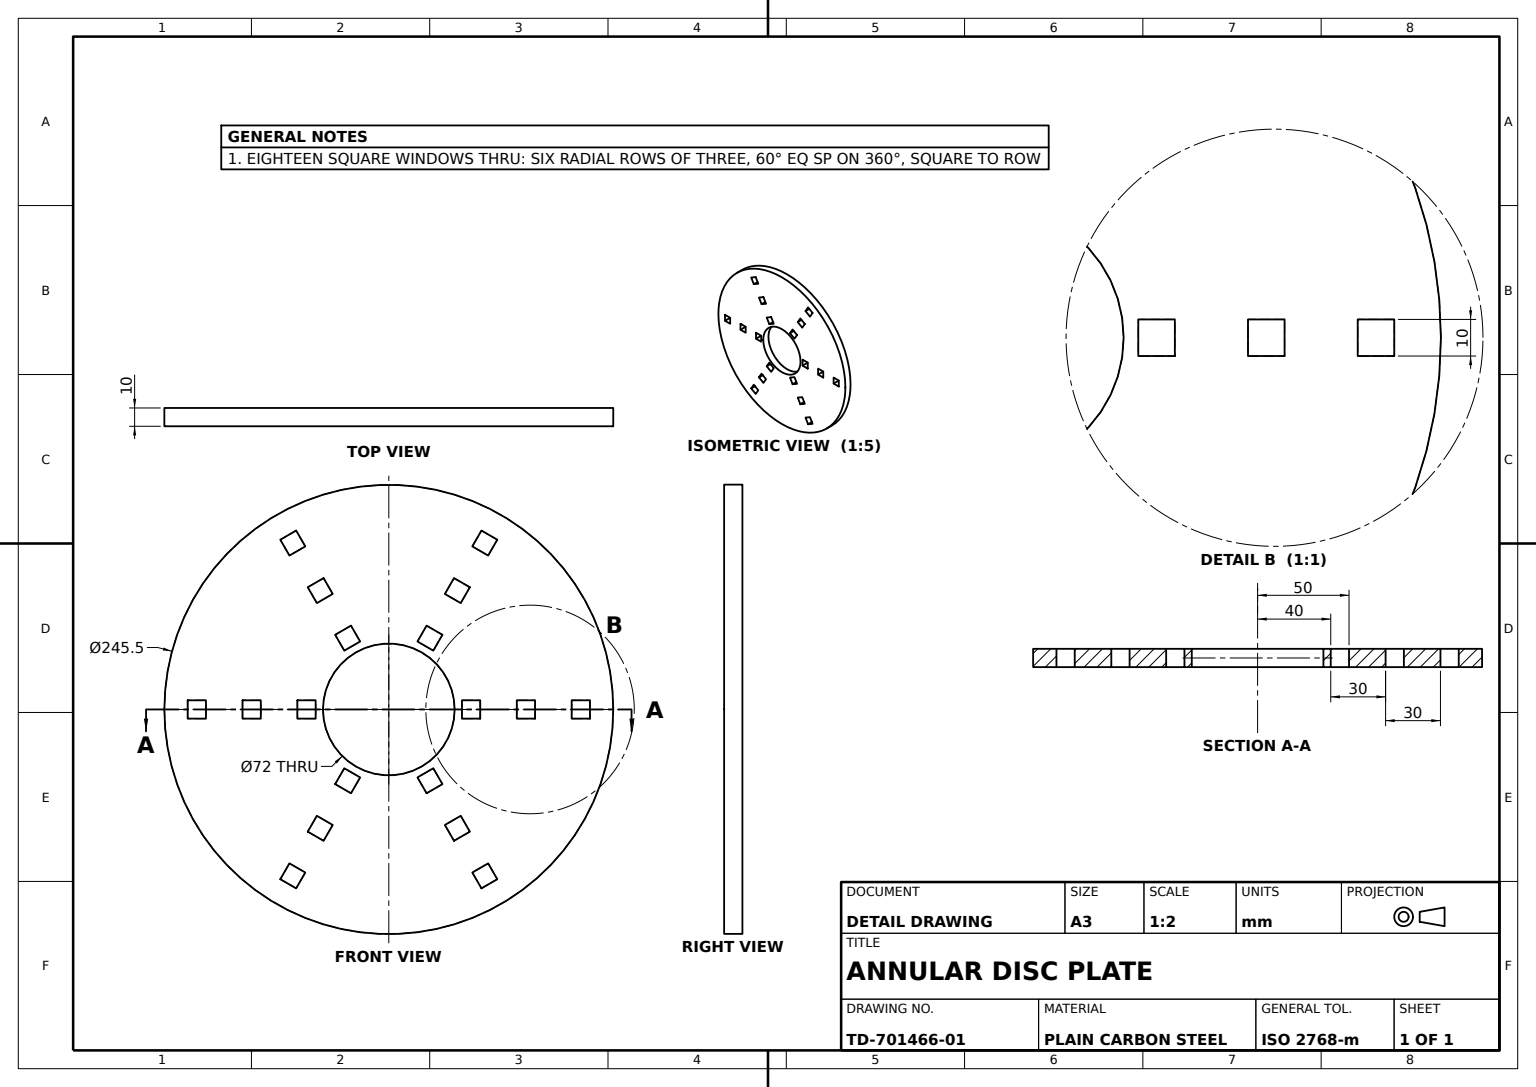
solid
v1 (54.330127,84.10254,10)
v2 (59.330127,92.762794,10)
e1 v1 v2 LINE
v3 (59.330127,92.762794,0)
e2 v3 v2 LINE
v4 (54.330127,84.10254,0)
e3 v4 v3 LINE
e4 v4 v1 LINE
face PLANE(AX(P(34.330127,49.461524,0),D(0.866025404,-0.5,0),D(0.5,0.866025404,0))) rev [e1 -e2 -e3 e4]
v5 (39.330127,-58.121778,0)
v6 (39.330127,-58.121778,10)
e5 v5 v6 LINE
v7 (30.669873,-63.121778,10)
e6 v7 v6 LINE
v8 (30.669873,-63.121778,0)
e7 v8 v7 LINE
e8 v8 v5 LINE
face PLANE(AX(P(35,-60.621778,0),D(0.5,-0.866025404,0),D(0.866025404,0.5,0))) [e5 -e6 -e7 e8]
v9 (29.330127,40.80127,0)
v10 (20.669873,45.80127,0)
e9 v9 v10 LINE
v11 (29.330127,40.80127,10)
e10 v9 v11 LINE
v12 (20.669873,45.80127,10)
e11 v11 v12 LINE
e12 v10 v12 LINE
face PLANE(AX(P(25,43.30127,0),D(0.5,0.866025404,0),D(-0.866025404,0.5,0))) rev [-e9 e10 e11 -e12]
v13 (-54.330127,-84.10254,0)
v14 (-45.669873,-89.10254,0)
e13 v13 v14 LINE
v15 (-45.669873,-89.10254,10)
e14 v14 v15 LINE
v16 (-54.330127,-84.10254,10)
e15 v16 v15 LINE
e16 v13 v16 LINE
face PLANE(AX(P(-50,-86.60254,0),D(-0.5,-0.866025404,0),D(0.866025404,-0.5,0))) [e13 e14 -e15 -e16]
v17 (122.75,0,10)
v18 (-122.75,0,10)
e17 v17 v18 CIRCLE(AX(P(0,0,10),D(0,0,1),D(1,0,0)),122.75)
e18 v18 v17 CIRCLE(AX(P(0,0,10),D(0,0,1),D(1,0,0)),122.75)
v19 (-15.669873,37.141016,10)
v20 (-24.330127,32.141016,10)
e19 v19 v20 LINE
v21 (-29.330127,40.80127,10)
e20 v21 v20 LINE
v22 (-20.669873,45.80127,10)
e21 v22 v21 LINE
e22 v19 v22 LINE
v23 (44.330127,66.782032,10)
v24 (35.669873,71.782032,10)
e23 v23 v24 LINE
v25 (39.330127,58.121778,10)
e24 v25 v23 LINE
v26 (30.669873,63.121778,10)
e25 v25 v26 LINE
e26 v24 v26 LINE
v27 (24.330127,32.141016,10)
e27 v27 v11 LINE
v28 (15.669873,37.141016,10)
e28 v27 v28 LINE
e29 v12 v28 LINE
v29 (-24.330127,-32.141016,10)
v30 (-15.669873,-37.141016,10)
e30 v29 v30 LINE
v31 (-20.669873,-45.80127,10)
e31 v31 v30 LINE
v32 (-29.330127,-40.80127,10)
e32 v32 v31 LINE
e33 v29 v32 LINE
v33 (-40,5,10)
v34 (-50,5,10)
e34 v33 v34 LINE
v35 (-40,-5,10)
e35 v33 v35 LINE
v36 (-50,-5,10)
e36 v36 v35 LINE
e37 v34 v36 LINE
v37 (29.330127,-40.80127,10)
v38 (24.330127,-32.141016,10)
e38 v37 v38 LINE
v39 (20.669873,-45.80127,10)
e39 v39 v37 LINE
v40 (15.669873,-37.141016,10)
e40 v40 v39 LINE
e41 v40 v38 LINE
v41 (35.669873,-71.782032,10)
e42 v7 v41 LINE
v42 (44.330127,-66.782032,10)
e43 v42 v6 LINE
e44 v41 v42 LINE
v43 (-50.669873,-97.762794,10)
e45 v43 v15 LINE
v44 (-59.330127,-92.762794,10)
e46 v44 v43 LINE
e47 v16 v44 LINE
v45 (50,5,10)
v46 (40,5,10)
e48 v45 v46 LINE
v47 (50,-5,10)
e49 v47 v45 LINE
v48 (40,-5,10)
e50 v48 v47 LINE
e51 v48 v46 LINE
v49 (-44.330127,66.782032,10)
v50 (-39.330127,58.121778,10)
e52 v49 v50 LINE
v51 (-35.669873,71.782032,10)
e53 v51 v49 LINE
v52 (-30.669873,63.121778,10)
e54 v52 v51 LINE
e55 v52 v50 LINE
v53 (-36,0,10)
v54 (36,0,10)
e56 v53 v54 CIRCLE(AX(P(0,0,10),D(0,0,1),D(1,0,0)),36)
e57 v54 v53 CIRCLE(AX(P(0,0,10),D(0,0,1),D(1,0,0)),36)
v55 (-39.330127,-58.121778,10)
v56 (-44.330127,-66.782032,10)
e58 v55 v56 LINE
v57 (-30.669873,-63.121778,10)
e59 v55 v57 LINE
v58 (-35.669873,-71.782032,10)
e60 v58 v57 LINE
e61 v56 v58 LINE
v59 (-80,5,10)
v60 (-80,-5,10)
e62 v59 v60 LINE
v61 (-70,5,10)
e63 v61 v59 LINE
v62 (-70,-5,10)
e64 v61 v62 LINE
e65 v60 v62 LINE
v63 (-59.330127,92.762794,10)
v64 (-54.330127,84.10254,10)
e66 v63 v64 LINE
v65 (-50.669873,97.762794,10)
e67 v65 v63 LINE
v66 (-45.669873,89.10254,10)
e68 v66 v65 LINE
e69 v66 v64 LINE
v67 (100,-5,10)
v68 (100,5,10)
e70 v67 v68 LINE
v69 (110,5,10)
e71 v69 v68 LINE
v70 (110,-5,10)
e72 v70 v69 LINE
e73 v67 v70 LINE
v71 (-110,5,10)
v72 (-110,-5,10)
e74 v71 v72 LINE
v73 (-100,5,10)
e75 v73 v71 LINE
v74 (-100,-5,10)
e76 v73 v74 LINE
e77 v72 v74 LINE
v75 (45.669873,-89.10254,10)
v76 (54.330127,-84.10254,10)
e78 v75 v76 LINE
v77 (59.330127,-92.762794,10)
e79 v77 v76 LINE
v78 (50.669873,-97.762794,10)
e80 v78 v77 LINE
e81 v75 v78 LINE
v79 (80,5,10)
v80 (70,5,10)
e82 v79 v80 LINE
v81 (80,-5,10)
e83 v81 v79 LINE
v82 (70,-5,10)
e84 v82 v81 LINE
e85 v82 v80 LINE
v83 (50.669873,97.762794,10)
v84 (45.669873,89.10254,10)
e86 v83 v84 LINE
e87 v2 v83 LINE
e88 v1 v84 LINE
face PLANE(AX(P(0,0,10),D(0,0,1),D(1,0,0))) [e17 e18] [e19 -e20 -e21 -e22] [-e23 -e24 e25 -e26] [-e11 -e27 e28 -e29] [e30 -e31 -e32 -e33] [-e34 e35 -e36 -e37] [-e38 -e39 -e40 e41] [-e42 e6 -e43 -e44] [-e45 -e46 -e47 e15] [-e48 -e49 -e50 e51] [-e52 -e53 -e54 e55] [-e56 -e57] [-e58 e59 -e60 -e61] [-e62 -e63 e64 -e65] [-e66 -e67 -e68 e69] [e70 -e71 -e72 -e73] [-e74 -e75 e76 -e77] [e78 -e79 -e80 -e81] [-e82 -e83 -e84 e85] [-e86 -e87 -e1 e88]
v85 (-36,0,0)
e89 v85 v53 LINE
v86 (36,0,0)
e90 v86 v54 LINE
e91 v85 v86 CIRCLE(AX(P(0,0,0),D(0,0,1),D(1,0,0)),36)
face CYL(AX(P(0,0,0),D(0,0,1),D(1,0,0)),36) rev [e89 e56 -e90 -e91]
v87 (29.330127,-40.80127,0)
e92 v87 v37 LINE
v88 (24.330127,-32.141016,0)
e93 v88 v38 LINE
e94 v87 v88 LINE
face PLANE(AX(P(4.330127,2.5,0),D(0.866025404,0.5,0),D(-0.5,0.866025404,0))) rev [e92 e38 -e93 -e94]
v89 (-35.669873,-71.782032,0)
v90 (-30.669873,-63.121778,0)
e95 v89 v90 LINE
e96 v89 v58 LINE
e97 v90 v57 LINE
face PLANE(AX(P(-10.669873,-28.480762,0),D(0.866025404,-0.5,0),D(0.5,0.866025404,0))) rev [-e95 e96 e60 -e97]
e98 v86 v85 CIRCLE(AX(P(0,0,0),D(0,0,1),D(1,0,0)),36)
face CYL(AX(P(0,0,0),D(0,0,1),D(1,0,0)),36) rev [-e98 e90 e57 -e89]
v91 (-45.669873,89.10254,0)
v92 (-50.669873,97.762794,0)
e99 v91 v92 LINE
e100 v91 v66 LINE
e101 v92 v65 LINE
face PLANE(AX(P(-25.669873,54.461524,0),D(0.866025404,0.5,0),D(-0.5,0.866025404,0))) rev [-e99 e100 e68 -e101]
v93 (35.669873,-71.782032,0)
e102 v8 v93 LINE
e103 v93 v41 LINE
face PLANE(AX(P(10.669873,-28.480762,0),D(-0.866025404,-0.5,0),D(0.5,-0.866025404,0))) rev [-e102 e7 e42 -e103]
v94 (20.669873,-45.80127,0)
e104 v94 v39 LINE
e105 v94 v87 LINE
face PLANE(AX(P(25,-43.30127,0),D(0.5,-0.866025404,0),D(0.866025404,0.5,0))) rev [e104 e39 -e92 -e105]
v95 (50,5,0)
e106 v95 v45 LINE
v96 (40,5,0)
e107 v96 v46 LINE
e108 v95 v96 LINE
face PLANE(AX(P(0,5,0),D(0,1,0),D(-1,0,0))) rev [e106 e48 -e107 -e108]
v97 (45.669873,-89.10254,0)
v98 (50.669873,-97.762794,0)
e109 v97 v98 LINE
e110 v97 v75 LINE
e111 v98 v78 LINE
face PLANE(AX(P(25.669873,-54.461524,0),D(-0.866025404,-0.5,0),D(0.5,-0.866025404,0))) rev [-e109 e110 e81 -e111]
v99 (50,-5,0)
e112 v99 v95 LINE
e113 v99 v47 LINE
face PLANE(AX(P(50,0,0),D(1,0,0),D(0,0,-1))) rev [-e106 -e112 e113 e49]
v100 (-40,-5,0)
e114 v100 v35 LINE
v101 (-50,-5,0)
e115 v101 v100 LINE
e116 v101 v36 LINE
face PLANE(AX(P(0,-5,0),D(0,-1,0),D(1,0,0))) rev [e36 -e114 -e115 e116]
v102 (35.669873,71.782032,0)
e117 v102 v24 LINE
v103 (44.330127,66.782032,0)
e118 v103 v102 LINE
e119 v103 v23 LINE
face PLANE(AX(P(40,69.282032,0),D(0.5,0.866025404,0),D(-0.866025404,0.5,0))) rev [e23 -e117 -e118 e119]
v104 (-39.330127,58.121778,0)
e120 v104 v50 LINE
v105 (-44.330127,66.782032,0)
e121 v105 v104 LINE
e122 v105 v49 LINE
face PLANE(AX(P(-19.330127,23.480762,0),D(-0.866025404,-0.5,0),D(0.5,-0.866025404,0))) rev [e52 -e120 -e121 e122]
v106 (39.330127,58.121778,0)
v107 (30.669873,63.121778,0)
e123 v106 v107 LINE
e124 v107 v26 LINE
e125 v106 v25 LINE
face PLANE(AX(P(35,60.621778,0),D(0.5,0.866025404,0),D(-0.866025404,0.5,0))) [e123 e124 -e25 -e125]
v108 (-110,-5,0)
v109 (-100,-5,0)
e126 v108 v109 LINE
e127 v108 v72 LINE
e128 v109 v74 LINE
face PLANE(AX(P(-60,-5,0),D(0,-1,0),D(1,0,0))) rev [-e126 e127 e77 -e128]
v110 (-100,5,0)
v111 (-110,5,0)
e129 v110 v111 LINE
e130 v110 v73 LINE
e131 v111 v71 LINE
face PLANE(AX(P(-60,5,0),D(0,1,0),D(0,0,1))) rev [-e129 e130 e75 -e131]
e132 v106 v103 LINE
face PLANE(AX(P(19.330127,23.480762,0),D(0.866025404,-0.5,0),D(0.5,0.866025404,0))) rev [e125 e24 -e119 -e132]
v112 (44.330127,-66.782032,0)
e133 v112 v42 LINE
e134 v112 v5 LINE
face PLANE(AX(P(19.330127,-23.480762,0),D(0.866025404,0.5,0),D(-0.5,0.866025404,0))) rev [e133 e43 -e5 -e134]
v113 (-50.669873,-97.762794,0)
e135 v113 v43 LINE
v114 (-59.330127,-92.762794,0)
e136 v114 v113 LINE
e137 v114 v44 LINE
face PLANE(AX(P(-55,-95.262794,0),D(-0.5,-0.866025404,0),D(0.866025404,-0.5,0))) rev [e46 -e135 -e136 e137]
v115 (-40,5,0)
e138 v115 v100 LINE
e139 v115 v33 LINE
face PLANE(AX(P(-40,0,0),D(-1,0,0),D(0,0,1))) [e138 e114 -e35 -e139]
v116 (100,-5,0)
v117 (100,5,0)
e140 v116 v117 LINE
e141 v117 v68 LINE
e142 v116 v67 LINE
face PLANE(AX(P(100,0,0),D(1,0,0),D(0,0,-1))) [e140 e141 -e70 -e142]
v118 (-122.75,0,0)
e143 v18 v118 LINE
v119 (122.75,0,0)
e144 v118 v119 CIRCLE(AX(P(0,0,0),D(0,0,1),D(1,0,0)),122.75)
e145 v17 v119 LINE
face CYL(AX(P(0,0,10),D(0,0,-1),D(-1,0,0)),122.75) [-e18 e143 e144 -e145]
v120 (-29.330127,40.80127,0)
e146 v120 v21 LINE
v121 (-20.669873,45.80127,0)
e147 v121 v120 LINE
e148 v121 v22 LINE
face PLANE(AX(P(-25,43.30127,0),D(-0.5,0.866025404,0),D(-0.866025404,-0.5,0))) rev [-e146 -e147 e148 e21]
e149 v110 v109 LINE
face PLANE(AX(P(-100,0,0),D(-1,0,0),D(0,0,1))) [e128 -e76 -e130 e149]
e150 v119 v118 CIRCLE(AX(P(0,0,0),D(0,0,1),D(1,0,0)),122.75)
face CYL(AX(P(0,0,10),D(0,0,-1),D(-1,0,0)),122.75) [e145 e150 -e143 -e17]
v122 (70,-5,0)
e151 v122 v82 LINE
v123 (70,5,0)
e152 v122 v123 LINE
e153 v123 v80 LINE
face PLANE(AX(P(70,0,0),D(1,0,0),D(0,0,-1))) [-e85 -e151 e152 e153]
e154 v111 v108 LINE
face PLANE(AX(P(-110,0,0),D(-1,0,0),D(0,0,1))) rev [-e127 -e154 e131 e74]
v124 (-80,-5,0)
e155 v124 v60 LINE
v125 (-80,5,0)
e156 v125 v124 LINE
e157 v125 v59 LINE
face PLANE(AX(P(-80,0,0),D(-1,0,0),D(0,0,1))) rev [e62 -e155 -e156 e157]
v126 (15.669873,-37.141016,0)
e158 v126 v40 LINE
e159 v126 v88 LINE
face PLANE(AX(P(20,-34.641016,0),D(0.5,-0.866025404,0),D(0.866025404,0.5,0))) [-e41 -e158 e159 e93]
v127 (-30.669873,63.121778,0)
e160 v127 v52 LINE
v128 (-35.669873,71.782032,0)
e161 v128 v51 LINE
e162 v127 v128 LINE
face PLANE(AX(P(-10.669873,28.480762,0),D(0.866025404,0.5,0),D(-0.5,0.866025404,0))) rev [e160 e54 -e161 -e162]
v129 (-50,5,0)
e163 v129 v101 LINE
e164 v129 v34 LINE
face PLANE(AX(P(-50,0,0),D(-1,0,0),D(0,0,1))) rev [e37 -e116 -e163 e164]
v130 (80,-5,0)
e165 v122 v130 LINE
e166 v130 v81 LINE
face PLANE(AX(P(30,-5,0),D(0,-1,0),D(0,0,-1))) rev [-e165 e151 e84 -e166]
e167 v127 v104 LINE
face PLANE(AX(P(-35,60.621778,0),D(-0.5,0.866025404,0),D(-0.866025404,-0.5,0))) [-e55 -e160 e167 e120]
v131 (59.330127,-92.762794,0)
e168 v131 v77 LINE
e169 v98 v131 LINE
face PLANE(AX(P(55,-95.262794,0),D(0.5,-0.866025404,0),D(0.866025404,0.5,0))) rev [e80 -e168 -e169 e111]
v132 (80,5,0)
e170 v130 v132 LINE
e171 v132 v79 LINE
face PLANE(AX(P(80,0,0),D(1,0,0),D(0,0,-1))) rev [-e170 e166 e83 -e171]
v133 (-39.330127,-58.121778,0)
e172 v133 v90 LINE
e173 v133 v55 LINE
face PLANE(AX(P(-35,-60.621778,0),D(-0.5,-0.866025404,0),D(0.866025404,-0.5,0))) [e172 e97 -e59 -e173]
v134 (50.669873,97.762794,0)
v135 (45.669873,89.10254,0)
e174 v134 v135 LINE
e175 v134 v83 LINE
e176 v135 v84 LINE
face PLANE(AX(P(25.669873,54.461524,0),D(-0.866025404,0.5,0),D(-0.5,-0.866025404,0))) rev [-e174 e175 e86 -e176]
v136 (-29.330127,-40.80127,0)
e177 v136 v32 LINE
v137 (-20.669873,-45.80127,0)
e178 v137 v31 LINE
e179 v136 v137 LINE
face PLANE(AX(P(-25,-43.30127,0),D(-0.5,-0.866025404,0),D(0.866025404,-0.5,0))) rev [e177 e32 -e178 -e179]
v138 (-70,5,0)
v139 (-70,-5,0)
e180 v138 v139 LINE
e181 v139 v62 LINE
e182 v138 v61 LINE
face PLANE(AX(P(-70,0,0),D(-1,0,0),D(0,0,1))) [e180 e181 -e64 -e182]
v140 (110,5,0)
e183 v140 v69 LINE
v141 (110,-5,0)
e184 v141 v140 LINE
e185 v141 v70 LINE
face PLANE(AX(P(110,0,0),D(1,0,0),D(0,0,-1))) rev [-e183 -e184 e185 e72]
v142 (-15.669873,37.141016,0)
e186 v142 v121 LINE
e187 v142 v19 LINE
face PLANE(AX(P(4.330127,2.5,0),D(0.866025404,0.5,0),D(-0.5,0.866025404,0))) rev [-e186 e187 e22 -e148]
e188 v4 v135 LINE
face PLANE(AX(P(50,86.60254,0),D(0.5,0.866025404,0),D(-0.866025404,0.5,0))) [e188 e176 -e88 -e4]
v143 (15.669873,37.141016,0)
e189 v143 v28 LINE
e190 v10 v143 LINE
face PLANE(AX(P(-4.330127,2.5,0),D(-0.866025404,0.5,0),D(-0.5,-0.866025404,0))) rev [e12 e29 -e189 -e190]
v144 (-24.330127,32.141016,0)
e191 v144 v20 LINE
e192 v120 v144 LINE
face PLANE(AX(P(-4.330127,-2.5,0),D(-0.866025404,-0.5,0),D(0.5,-0.866025404,0))) rev [-e191 -e192 e146 e20]
e193 v102 v107 LINE
face PLANE(AX(P(10.669873,28.480762,0),D(-0.866025404,0.5,0),D(-0.5,-0.866025404,0))) rev [-e124 -e193 e117 e26]
v145 (-59.330127,92.762794,0)
e194 v92 v145 LINE
e195 v145 v63 LINE
face PLANE(AX(P(-55,95.262794,0),D(-0.5,0.866025404,0),D(-0.866025404,-0.5,0))) rev [-e194 e101 e67 -e195]
v146 (40,-5,0)
e196 v146 v48 LINE
e197 v146 v99 LINE
face PLANE(AX(P(0,-5,0),D(0,-1,0),D(0,0,-1))) rev [e196 e50 -e113 -e197]
e198 v115 v129 LINE
face PLANE(AX(P(0,5,0),D(0,1,0),D(0,0,1))) rev [e139 e34 -e164 -e198]
v147 (-54.330127,84.10254,0)
e199 v91 v147 LINE
e200 v147 v64 LINE
face PLANE(AX(P(-50,86.60254,0),D(-0.5,0.866025404,0),D(-0.866025404,-0.5,0))) [e199 e200 -e69 -e100]
e201 v142 v144 LINE
face PLANE(AX(P(-20,34.641016,0),D(-0.5,0.866025404,0),D(-0.866025404,-0.5,0))) [e201 e191 -e19 -e187]
v148 (-15.669873,-37.141016,0)
e202 v137 v148 LINE
e203 v148 v30 LINE
face PLANE(AX(P(4.330127,-2.5,0),D(0.866025404,-0.5,0),D(0.5,0.866025404,0))) rev [-e202 e178 e31 -e203]
v149 (-24.330127,-32.141016,0)
e204 v149 v29 LINE
e205 v149 v148 LINE
face PLANE(AX(P(-20,-34.641016,0),D(-0.5,-0.866025404,0),D(0.866025404,-0.5,0))) [-e30 -e204 e205 e203]
e206 v145 v147 LINE
face PLANE(AX(P(-34.330127,49.461524,0),D(-0.866025404,-0.5,0),D(0.5,-0.866025404,0))) rev [-e206 e195 e66 -e200]
e207 v128 v105 LINE
face PLANE(AX(P(-40,69.282032,0),D(-0.5,0.866025404,0),D(-0.866025404,-0.5,0))) rev [e53 -e122 -e207 e161]
e208 v13 v114 LINE
face PLANE(AX(P(-34.330127,-49.461524,0),D(-0.866025404,0.5,0),D(-0.5,-0.866025404,0))) rev [e47 -e137 -e208 e16]
e209 v149 v136 LINE
face PLANE(AX(P(-4.330127,2.5,0),D(-0.866025404,0.5,0),D(-0.5,-0.866025404,0))) rev [-e177 -e209 e204 e33]
v150 (-44.330127,-66.782032,0)
e210 v150 v56 LINE
e211 v133 v150 LINE
face PLANE(AX(P(-19.330127,-23.480762,0),D(-0.866025404,0.5,0),D(-0.5,-0.866025404,0))) rev [e173 e58 -e210 -e211]
e212 v150 v89 LINE
face PLANE(AX(P(-40,-69.282032,0),D(-0.5,-0.866025404,0),D(0.866025404,-0.5,0))) rev [-e96 -e212 e210 e61]
v151 (24.330127,32.141016,0)
e213 v151 v9 LINE
e214 v151 v27 LINE
face PLANE(AX(P(4.330127,-2.5,0),D(0.866025404,-0.5,0),D(0.5,0.866025404,0))) rev [-e10 -e213 e214 e27]
v152 (54.330127,-84.10254,0)
e215 v152 v76 LINE
e216 v131 v152 LINE
face PLANE(AX(P(34.330127,-49.461524,0),D(0.866025404,0.5,0),D(-0.5,0.866025404,0))) rev [e79 -e215 -e216 e168]
e217 v93 v112 LINE
face PLANE(AX(P(40,-69.282032,0),D(0.5,-0.866025404,0),D(0.866025404,0.5,0))) rev [e103 e44 -e133 -e217]
e218 v140 v117 LINE
face PLANE(AX(P(60,5,0),D(0,1,0),D(-1,0,0))) rev [e183 e71 -e141 -e218]
e219 v113 v14 LINE
face PLANE(AX(P(-25.669873,-54.461524,0),D(0.866025404,-0.5,0),D(0.5,0.866025404,0))) rev [-e219 e135 e45 -e14]
e220 v151 v143 LINE
face PLANE(AX(P(20,34.641016,0),D(0.5,0.866025404,0),D(-0.866025404,0.5,0))) [e189 -e28 -e214 e220]
e221 v124 v139 LINE
face PLANE(AX(P(-30,-5,0),D(0,-1,0),D(1,0,0))) rev [e155 e65 -e181 -e221]
e222 v97 v152 LINE
face PLANE(AX(P(50,-86.60254,0),D(0.5,-0.866025404,0),D(0.866025404,0.5,0))) [e215 -e78 -e110 e222]
e223 v146 v96 LINE
e224 v126 v94 LINE
e225 v132 v123 LINE
e226 v116 v141 LINE
e227 v138 v125 LINE
e228 v3 v134 LINE
face PLANE(AX(P(0,0,0),D(0,0,1),D(1,0,0))) rev [e118 e193 -e123 e132] [e207 e121 -e167 e162] [e212 e95 -e172 e211] [e202 -e205 e209 e179] [e126 -e149 e129 e154] [e192 -e201 e186 e147] [e109 e169 e216 -e222] [e112 e108 -e223 e197] [-e159 e224 e105 e94] [e163 e115 -e138 e198] [e208 e136 e219 -e13] [e165 e170 e225 -e152] [e99 e194 e206 -e199] [e190 -e220 e213 e9] [-e8 e102 e217 e134] [-e140 e226 e184 e218] [e227 e156 e221 -e180] [e98 e91] [e174 -e188 e3 e228] [-e144 -e150]
face PLANE(AX(P(55,95.262794,0),D(0.5,0.866025404,0),D(-0.866025404,0.5,0))) rev [-e228 e2 e87 -e175]
face PLANE(AX(P(-4.330127,-2.5,0),D(-0.866025404,-0.5,0),D(0.5,-0.866025404,0))) rev [-e224 e158 e40 -e104]
face PLANE(AX(P(-30,5,0),D(0,1,0),D(0,0,1))) rev [e63 -e157 -e227 e182]
face PLANE(AX(P(40,0,0),D(1,0,0),D(0,0,-1))) [e107 -e51 -e196 e223]
face PLANE(AX(P(30,5,0),D(0,1,0),D(-1,0,0))) rev [e82 -e153 -e225 e171]
face PLANE(AX(P(60,-5,0),D(0,-1,0),D(0,0,-1))) rev [e142 e73 -e185 -e226]
